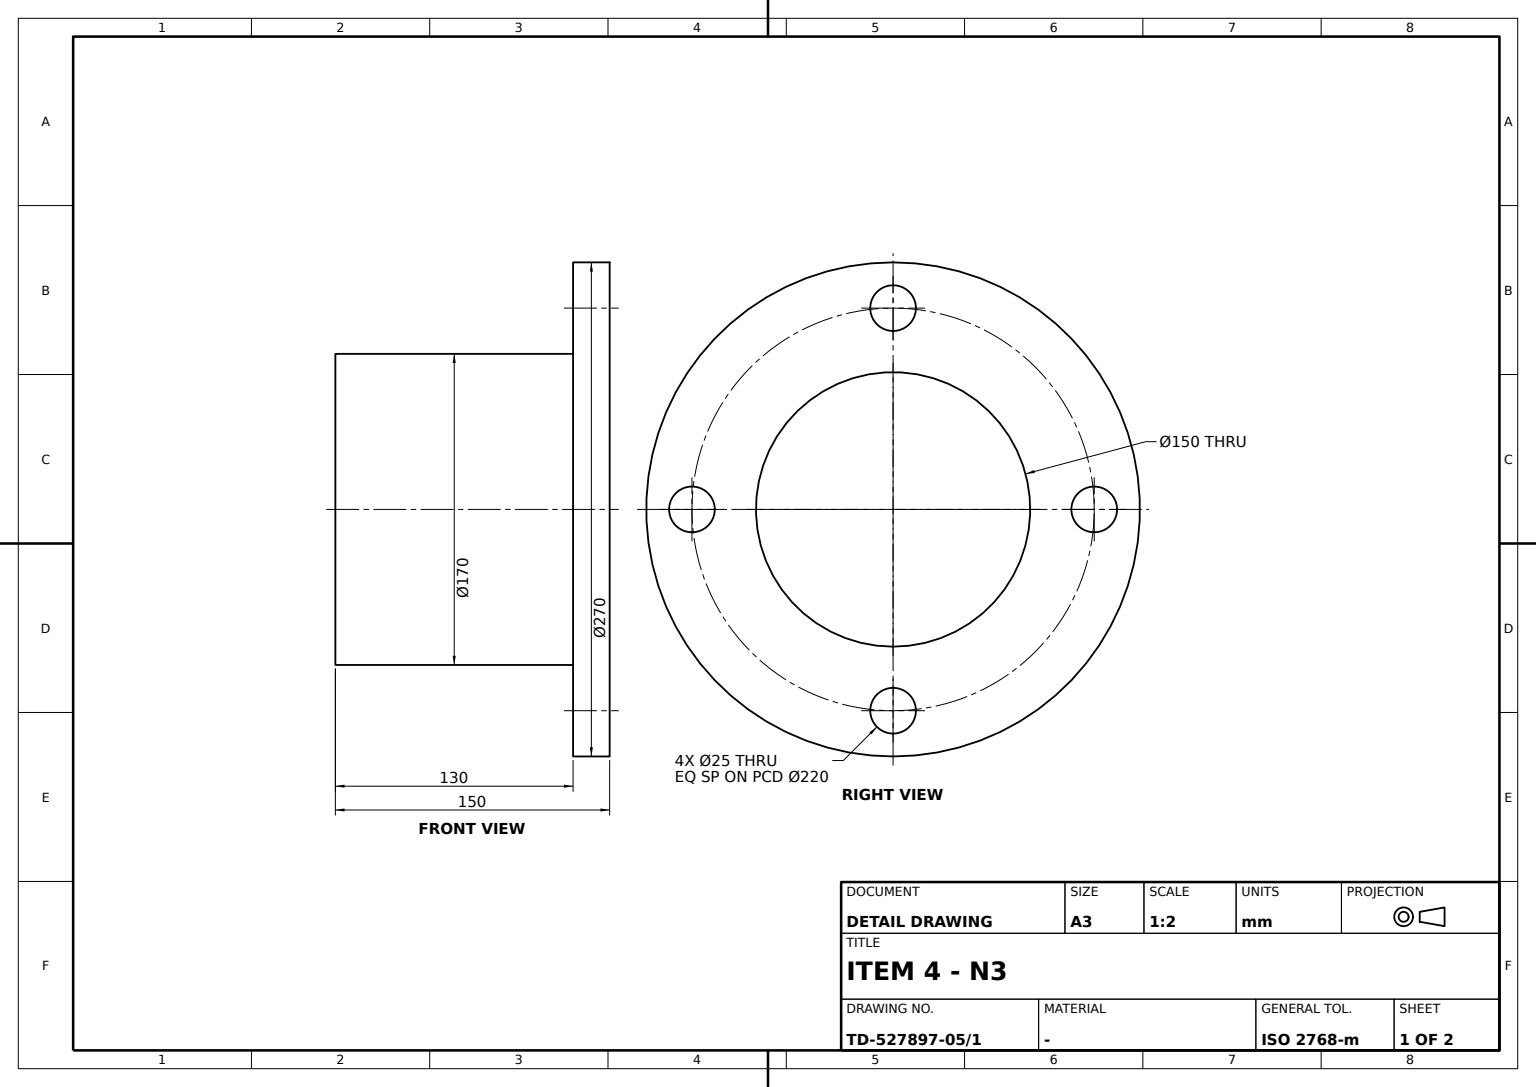
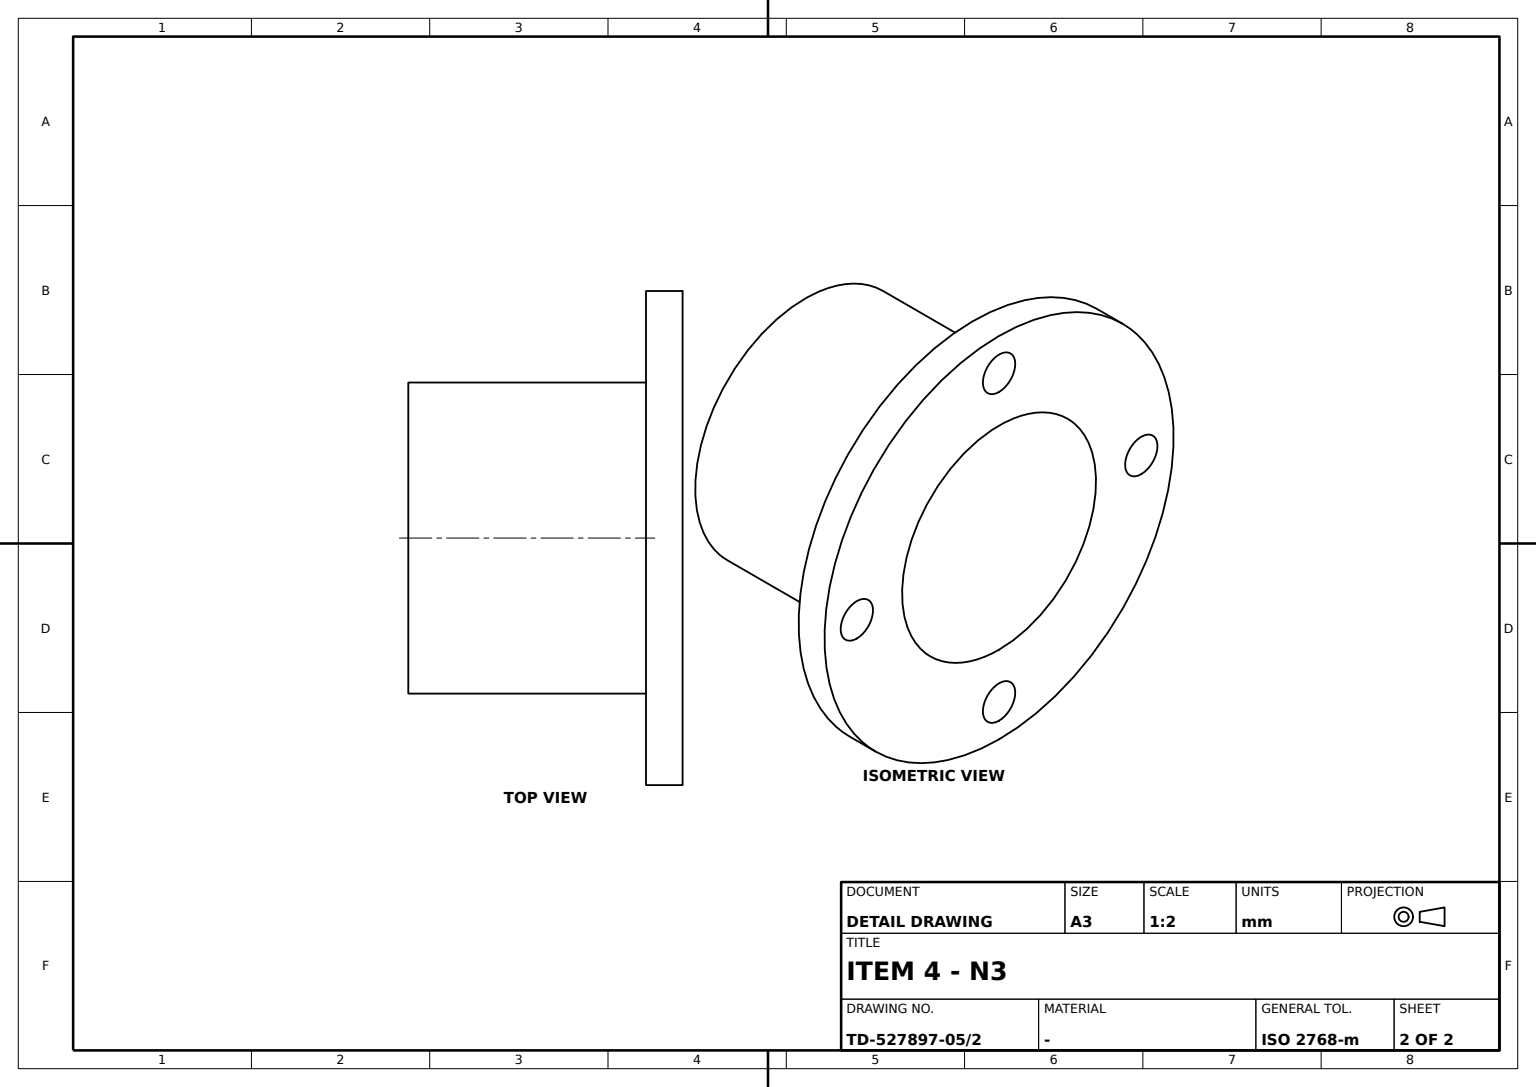
ISO-10303-21;
HEADER;
FILE_DESCRIPTION((''),'2;1');
FILE_NAME('','',(''),(''),'','','');
FILE_SCHEMA(('AUTOMOTIVE_DESIGN'));
ENDSEC;
DATA;
#1=APPLICATION_CONTEXT('');
#2=PRODUCT_CONTEXT('',#1,'mechanical');
#3=PRODUCT('','','',(#2));
#4=PRODUCT_DEFINITION_FORMATION('','',#3);
#5=PRODUCT_DEFINITION_CONTEXT('',#1,'design');
#6=PRODUCT_DEFINITION('','',#4,#5);
#7=PRODUCT_DEFINITION_SHAPE('','',#6);
#8=(LENGTH_UNIT()NAMED_UNIT(*)SI_UNIT(.MILLI.,.METRE.));
#9=(NAMED_UNIT(*)PLANE_ANGLE_UNIT()SI_UNIT($,.RADIAN.));
#10=(NAMED_UNIT(*)SI_UNIT($,.STERADIAN.)SOLID_ANGLE_UNIT());
#11=UNCERTAINTY_MEASURE_WITH_UNIT(LENGTH_MEASURE(0.005),#8,'distance_accuracy_value','');
#12=(GEOMETRIC_REPRESENTATION_CONTEXT(3)GLOBAL_UNCERTAINTY_ASSIGNED_CONTEXT((#11))GLOBAL_UNIT_ASSIGNED_CONTEXT((#8,#9,#10))REPRESENTATION_CONTEXT('',''));
#13=CARTESIAN_POINT('',(1212.5,-1310.,2630.));
#14=VERTEX_POINT('',#13);
#15=CARTESIAN_POINT('',(1200.,-1310.,2630.));
#16=DIRECTION('',(0.,0.,1.));
#17=DIRECTION('',(1.,0.,0.));
#18=AXIS2_PLACEMENT_3D('',#15,#16,#17);
#19=CIRCLE('',#18,12.5);
#20=EDGE_CURVE('',#14,#14,#19,.T.);
#21=ORIENTED_EDGE('',*,*,#20,.F.);
#22=EDGE_LOOP('',(#21));
#23=FACE_BOUND('',#22,.T.);
#24=CARTESIAN_POINT('',(1212.5,-1310.,2650.));
#25=VERTEX_POINT('',#24);
#26=CARTESIAN_POINT('',(1200.,-1310.,2650.));
#27=AXIS2_PLACEMENT_3D('',#26,#16,#17);
#28=CIRCLE('',#27,12.5);
#29=EDGE_CURVE('',#25,#25,#28,.T.);
#30=ORIENTED_EDGE('',*,*,#29,.T.);
#31=EDGE_LOOP('',(#30));
#32=FACE_BOUND('',#31,.T.);
#33=CARTESIAN_POINT('',(1200.,-1310.,2640.));
#34=AXIS2_PLACEMENT_3D('',#33,#16,#17);
#35=CYLINDRICAL_SURFACE('',#34,12.5);
#36=ADVANCED_FACE('',(#23,#32),#35,.F.);
#37=CARTESIAN_POINT('',(1285.,-1200.,2500.));
#38=VERTEX_POINT('',#37);
#39=CARTESIAN_POINT('',(1200.,-1200.,2500.));
#40=AXIS2_PLACEMENT_3D('',#39,#16,#17);
#41=CIRCLE('',#40,85.);
#42=EDGE_CURVE('',#38,#38,#41,.T.);
#43=ORIENTED_EDGE('',*,*,#42,.T.);
#44=EDGE_LOOP('',(#43));
#45=FACE_BOUND('',#44,.T.);
#46=CARTESIAN_POINT('',(1285.,-1200.,2630.));
#47=VERTEX_POINT('',#46);
#48=CARTESIAN_POINT('',(1200.,-1200.,2630.));
#49=AXIS2_PLACEMENT_3D('',#48,#16,#17);
#50=CIRCLE('',#49,85.);
#51=EDGE_CURVE('',#47,#47,#50,.T.);
#52=ORIENTED_EDGE('',*,*,#51,.F.);
#53=EDGE_LOOP('',(#52));
#54=FACE_BOUND('',#53,.T.);
#55=CARTESIAN_POINT('',(1200.,-1200.,2575.));
#56=AXIS2_PLACEMENT_3D('',#55,#16,#17);
#57=CYLINDRICAL_SURFACE('',#56,85.);
#58=ADVANCED_FACE('',(#45,#54),#57,.T.);
#59=CARTESIAN_POINT('',(1335.,-1200.,2630.));
#60=VERTEX_POINT('',#59);
#61=CIRCLE('',#49,135.);
#62=EDGE_CURVE('',#60,#60,#61,.T.);
#63=ORIENTED_EDGE('',*,*,#62,.T.);
#64=EDGE_LOOP('',(#63));
#65=FACE_BOUND('',#64,.T.);
#66=CARTESIAN_POINT('',(1335.,-1200.,2650.));
#67=VERTEX_POINT('',#66);
#68=CARTESIAN_POINT('',(1200.,-1200.,2650.));
#69=AXIS2_PLACEMENT_3D('',#68,#16,#17);
#70=CIRCLE('',#69,135.);
#71=EDGE_CURVE('',#67,#67,#70,.T.);
#72=ORIENTED_EDGE('',*,*,#71,.F.);
#73=EDGE_LOOP('',(#72));
#74=FACE_BOUND('',#73,.T.);
#75=CARTESIAN_POINT('',(1200.,-1200.,2640.));
#76=AXIS2_PLACEMENT_3D('',#75,#16,#17);
#77=CYLINDRICAL_SURFACE('',#76,135.);
#78=ADVANCED_FACE('',(#65,#74),#77,.T.);
#79=ORIENTED_EDGE('',*,*,#20,.T.);
#80=EDGE_LOOP('',(#79));
#81=FACE_BOUND('',#80,.T.);
#82=ORIENTED_EDGE('',*,*,#51,.T.);
#83=EDGE_LOOP('',(#82));
#84=FACE_BOUND('',#83,.T.);
#85=ORIENTED_EDGE('',*,*,#62,.F.);
#86=EDGE_LOOP('',(#85));
#87=FACE_BOUND('',#86,.T.);
#88=CARTESIAN_POINT('',(1212.5,-1090.,2630.));
#89=VERTEX_POINT('',#88);
#90=CARTESIAN_POINT('',(1200.,-1090.,2630.));
#91=AXIS2_PLACEMENT_3D('',#90,#16,#17);
#92=CIRCLE('',#91,12.5);
#93=EDGE_CURVE('',#89,#89,#92,.T.);
#94=ORIENTED_EDGE('',*,*,#93,.T.);
#95=EDGE_LOOP('',(#94));
#96=FACE_BOUND('',#95,.T.);
#97=CARTESIAN_POINT('',(1322.5,-1200.,2630.));
#98=VERTEX_POINT('',#97);
#99=CARTESIAN_POINT('',(1310.,-1200.,2630.));
#100=AXIS2_PLACEMENT_3D('',#99,#16,#17);
#101=CIRCLE('',#100,12.5);
#102=EDGE_CURVE('',#98,#98,#101,.T.);
#103=ORIENTED_EDGE('',*,*,#102,.T.);
#104=EDGE_LOOP('',(#103));
#105=FACE_BOUND('',#104,.T.);
#106=CARTESIAN_POINT('',(1102.5,-1200.,2630.));
#107=VERTEX_POINT('',#106);
#108=CARTESIAN_POINT('',(1090.,-1200.,2630.));
#109=AXIS2_PLACEMENT_3D('',#108,#16,#17);
#110=CIRCLE('',#109,12.5);
#111=EDGE_CURVE('',#107,#107,#110,.T.);
#112=ORIENTED_EDGE('',*,*,#111,.T.);
#113=EDGE_LOOP('',(#112));
#114=FACE_BOUND('',#113,.T.);
#115=CARTESIAN_POINT('',(0.,0.,2630.));
#116=AXIS2_PLACEMENT_3D('',#115,#16,#17);
#117=PLANE('',#116);
#118=ADVANCED_FACE('',(#81,#84,#87,#96,#105,#114),#117,.F.);
#119=CARTESIAN_POINT('',(1322.5,-1200.,2650.));
#120=VERTEX_POINT('',#119);
#121=CARTESIAN_POINT('',(1310.,-1200.,2650.));
#122=AXIS2_PLACEMENT_3D('',#121,#16,#17);
#123=CIRCLE('',#122,12.5);
#124=EDGE_CURVE('',#120,#120,#123,.T.);
#125=ORIENTED_EDGE('',*,*,#124,.T.);
#126=EDGE_LOOP('',(#125));
#127=FACE_BOUND('',#126,.T.);
#128=ORIENTED_EDGE('',*,*,#102,.F.);
#129=EDGE_LOOP('',(#128));
#130=FACE_BOUND('',#129,.T.);
#131=CARTESIAN_POINT('',(1310.,-1200.,2640.));
#132=AXIS2_PLACEMENT_3D('',#131,#16,#17);
#133=CYLINDRICAL_SURFACE('',#132,12.5);
#134=ADVANCED_FACE('',(#127,#130),#133,.F.);
#135=CARTESIAN_POINT('',(1275.,-1200.,2650.));
#136=VERTEX_POINT('',#135);
#137=CIRCLE('',#69,75.);
#138=EDGE_CURVE('',#136,#136,#137,.T.);
#139=ORIENTED_EDGE('',*,*,#138,.F.);
#140=EDGE_LOOP('',(#139));
#141=FACE_BOUND('',#140,.T.);
#142=CARTESIAN_POINT('',(1102.5,-1200.,2650.));
#143=VERTEX_POINT('',#142);
#144=CARTESIAN_POINT('',(1090.,-1200.,2650.));
#145=AXIS2_PLACEMENT_3D('',#144,#16,#17);
#146=CIRCLE('',#145,12.5);
#147=EDGE_CURVE('',#143,#143,#146,.T.);
#148=ORIENTED_EDGE('',*,*,#147,.F.);
#149=EDGE_LOOP('',(#148));
#150=FACE_BOUND('',#149,.T.);
#151=ORIENTED_EDGE('',*,*,#124,.F.);
#152=EDGE_LOOP('',(#151));
#153=FACE_BOUND('',#152,.T.);
#154=ORIENTED_EDGE('',*,*,#71,.T.);
#155=EDGE_LOOP('',(#154));
#156=FACE_BOUND('',#155,.T.);
#157=ORIENTED_EDGE('',*,*,#29,.F.);
#158=EDGE_LOOP('',(#157));
#159=FACE_BOUND('',#158,.T.);
#160=CARTESIAN_POINT('',(1212.5,-1090.,2650.));
#161=VERTEX_POINT('',#160);
#162=CARTESIAN_POINT('',(1200.,-1090.,2650.));
#163=AXIS2_PLACEMENT_3D('',#162,#16,#17);
#164=CIRCLE('',#163,12.5);
#165=EDGE_CURVE('',#161,#161,#164,.T.);
#166=ORIENTED_EDGE('',*,*,#165,.F.);
#167=EDGE_LOOP('',(#166));
#168=FACE_BOUND('',#167,.T.);
#169=CARTESIAN_POINT('',(0.,0.,2650.));
#170=AXIS2_PLACEMENT_3D('',#169,#16,#17);
#171=PLANE('',#170);
#172=ADVANCED_FACE('',(#141,#150,#153,#156,#159,#168),#171,.T.);
#173=ORIENTED_EDGE('',*,*,#147,.T.);
#174=EDGE_LOOP('',(#173));
#175=FACE_BOUND('',#174,.T.);
#176=ORIENTED_EDGE('',*,*,#111,.F.);
#177=EDGE_LOOP('',(#176));
#178=FACE_BOUND('',#177,.T.);
#179=CARTESIAN_POINT('',(1090.,-1200.,2640.));
#180=AXIS2_PLACEMENT_3D('',#179,#16,#17);
#181=CYLINDRICAL_SURFACE('',#180,12.5);
#182=ADVANCED_FACE('',(#175,#178),#181,.F.);
#183=ORIENTED_EDGE('',*,*,#42,.F.);
#184=EDGE_LOOP('',(#183));
#185=FACE_BOUND('',#184,.T.);
#186=CARTESIAN_POINT('',(1275.,-1200.,2500.));
#187=VERTEX_POINT('',#186);
#188=CIRCLE('',#40,75.);
#189=EDGE_CURVE('',#187,#187,#188,.T.);
#190=ORIENTED_EDGE('',*,*,#189,.T.);
#191=EDGE_LOOP('',(#190));
#192=FACE_BOUND('',#191,.T.);
#193=CARTESIAN_POINT('',(0.,0.,2500.));
#194=AXIS2_PLACEMENT_3D('',#193,#16,#17);
#195=PLANE('',#194);
#196=ADVANCED_FACE('',(#185,#192),#195,.F.);
#197=ORIENTED_EDGE('',*,*,#165,.T.);
#198=EDGE_LOOP('',(#197));
#199=FACE_BOUND('',#198,.T.);
#200=ORIENTED_EDGE('',*,*,#93,.F.);
#201=EDGE_LOOP('',(#200));
#202=FACE_BOUND('',#201,.T.);
#203=CARTESIAN_POINT('',(1200.,-1090.,2640.));
#204=AXIS2_PLACEMENT_3D('',#203,#16,#17);
#205=CYLINDRICAL_SURFACE('',#204,12.5);
#206=ADVANCED_FACE('',(#199,#202),#205,.F.);
#207=ORIENTED_EDGE('',*,*,#189,.F.);
#208=EDGE_LOOP('',(#207));
#209=FACE_BOUND('',#208,.T.);
#210=ORIENTED_EDGE('',*,*,#138,.T.);
#211=EDGE_LOOP('',(#210));
#212=FACE_BOUND('',#211,.T.);
#213=CYLINDRICAL_SURFACE('',#56,75.);
#214=ADVANCED_FACE('',(#209,#212),#213,.F.);
#215=CLOSED_SHELL('',(#36,#58,#78,#118,#134,#172,#182,#196,#206,#214));
#216=MANIFOLD_SOLID_BREP('',#215);
#217=ADVANCED_BREP_SHAPE_REPRESENTATION('',(#216),#12);
#218=SHAPE_DEFINITION_REPRESENTATION(#7,#217);
ENDSEC;
END-ISO-10303-21;
